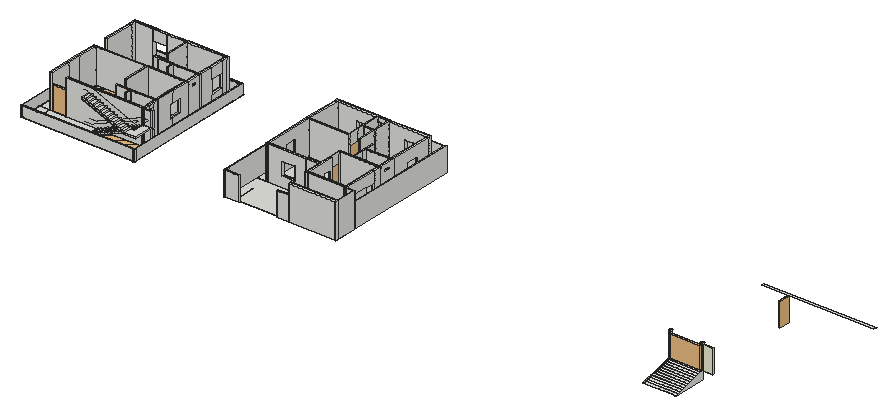
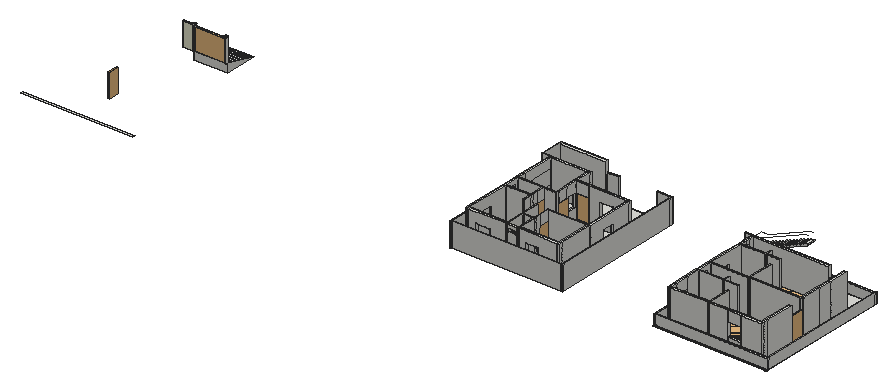
# SketchUp Ruby script. Lengths in inches.
U = 1.inch
M = Sketchup.active_model
def pt(a) = Geom::Point3d.new(a.map { |v| v * U })
def face(e, loops, mat)
  f = e.add_face(loops[0].map { |a| pt(a) })
  loops[1..].each { |l| e.add_face(l.map { |a| pt(a) }).erase! }
  f.material = f.back_material = mat if mat
  f
end
# faces: each face lists its corners as indices into pts; further lists are holes
def faces(e, pts, list, mat = nil) = list.each { |f| face(e, (f[0].is_a?(Array) ? f : [f]).map { |l| l.map { |i| pts[i] } }, mat) }
# xy, xz, yz: faces in a plane at the given z, y or x. An outline is a flat list of corners, or four numbers for a rectangle; further outlines are holes
def ring(l) = l.size == 4 ? [[l[0], l[1]], [l[2], l[1]], [l[2], l[3]], [l[0], l[3]]] : l.each_slice(2).to_a
def flat(e, list, mat, &to3) = list.each { |f| face(e, (f[0].is_a?(Array) ? f : [f]).map { |l| ring(l).map { |u, v| to3.(u, v) } }, mat) }
def xy(e, z, list, mat = nil) = flat(e, list, mat) { |x, y| [x, y, z] }
def xz(e, y, list, mat = nil) = flat(e, list, mat) { |x, z| [x, y, z] }
def yz(e, x, list, mat = nil) = flat(e, list, mat) { |y, z| [x, y, z] }
def lines(e, pts, list) = list.each { |a, b| e.add_line(pt(pts[a]), pt(pts[b])) }
# prism: a flat outline (further loops are holes) pulled along v
def prism(e, loops, v, mat = nil)
  f = face(e, loops, mat); d = Geom::Vector3d.new(v.map { |x| x * U })
  f.pushpull(f.normal.samedirection?(d) ? d.length : -d.length)
end
def box(e, o, s, mat = nil) = prism(e, [[o, [o[0] + s[0], o[1], o[2]], [o[0] + s[0], o[1] + s[1], o[2]], [o[0], o[1] + s[1], o[2]]]], [0, 0, s[2]], mat)
def at(x, y, z, deg = 0) = Geom::Transformation.translation(pt([x, y, z])) * Geom::Transformation.rotation(ORIGIN, Z_AXIS, deg.degrees)
def axes(o, x, y, z) = Geom::Transformation.new([*x, 0, *y, 0, *z, 0, *pt(o).to_a, 1])
def part(name) = M.definitions.add(name)
# library, detail: a bought-in or finely detailed component or shape, given as its bounding box
def library(name, o, s) = part(name).tap { |d| box(d.entities, o, s) }
def detail(e, o, s) = box(e.add_group.entities, o, s)
def put(e, d, t, mat = nil) = e.add_instance(d, t).tap { |i| i.material = mat if mat }
def group(e, t, mat = nil) = e.add_group.tap { |g| g.transformation = t; g.material = mat if mat }.entities
root = M.entities
M.materials.add("0001 AP 9436 AIR BREEZE").color = [243, 237, 232]
M.materials.add("0746 AP 7715 LUMINOUS").color = [235, 235, 209]
c1 = library("Group\#12",[0,0,0],[6.9375,42,86.5])
c2 = library("Group\#45",[0,0,0],[399.01,472.04,0.01])
c3 = part("Group\#29")
xy(c3.entities,0,[[0,0,0,179.49,176.02,179.49,176.02,89,180.99,89,180.99,179.49,311,179.49,311,53,176.02,53,176.02,47.99,222,47.99,222,30.01,227.01,30.01,227.01,47.99,311,47.99,311,0]])
c4 = part("Group19\#2")
p = [[1706.5625,247.76,0],[1706.5625,271.76,0],[1706.5625,427.76,65],[1706.5625,431.76,65],[1720.5625,431.76,65],[1720.5625,427.76,65],
  [1720.5625,283.76,125],[1720.5625,271.76,125],[1686.5625,247.76,0],[1686.5625,271.76,0],[1686.5625,427.76,65],[1686.5625,451.76,65],
  [1740.5625,451.76,65],[1740.5625,427.76,65],[1740.5625,283.76,125],[1740.5625,271.76,125]]
lines(c4.entities,p,[[0,1],[1,2],[2,3],[3,4],[4,5],[5,6],[6,7],[8,9],[9,10],[10,11],[11,12],[12,13],
  [13,14],[14,15]])
c5 = part("Group18\#3")
xy(c5.entities,-3.9375,[[1682.5625,271.76,1710.5625,283.76],[1682.5625,283.76,1710.5625,284.55]])
xy(c5.entities,0,[[1682.5625,271.76,1710.5625,283.76]])
xy(c5.entities,5,[[1682.5625,283.76,1710.5625,295.76]])
xy(c5.entities,10,[[1682.5625,295.76,1710.5625,307.76]])
xy(c5.entities,15,[[1682.5625,307.76,1710.5625,319.76]])
xy(c5.entities,20,[[1682.5625,319.76,1710.5625,331.76]])
xy(c5.entities,25,[[1682.5625,331.76,1710.5625,343.76]])
xy(c5.entities,30,[[1682.5625,343.76,1710.5625,355.76]])
xy(c5.entities,35,[[1682.5625,355.76,1710.5625,367.76]])
xy(c5.entities,40,[[1682.5625,367.76,1710.5625,379.76]])
xy(c5.entities,45,[[1682.5625,379.76,1710.5625,391.76]])
xy(c5.entities,50,[[1682.5625,391.76,1710.5625,403.76]])
xy(c5.entities,55,[[1682.5625,403.76,1710.5625,415.76]])
xy(c5.entities,60,[[1682.5625,415.76,1710.5625,427.76]])
xy(c5.entities,61.0625,[[1716.5625,414.97,1716.5625,427.76,1710.5625,427.76,1710.5625,440.55,1682.5625,440.55,1682.5625,455.76,1744.5625,455.76,1744.5625,414.97]])
xy(c5.entities,65,[[1716.5625,415.76,1744.5625,415.76,1744.5625,455.76,1682.5625,455.76,1682.5625,427.76,1716.5625,427.76]])
xy(c5.entities,70,[[1716.5625,403.76,1744.5625,415.76]])
xy(c5.entities,75,[[1716.5625,391.76,1744.5625,403.76]])
xy(c5.entities,80,[[1716.5625,379.76,1744.5625,391.76]])
xy(c5.entities,85,[[1716.5625,367.76,1744.5625,379.76]])
xy(c5.entities,90,[[1716.5625,355.76,1744.5625,367.76]])
xy(c5.entities,95,[[1716.5625,343.76,1744.5625,355.76]])
xy(c5.entities,100,[[1716.5625,331.76,1744.5625,343.76]])
xy(c5.entities,105,[[1716.5625,319.76,1744.5625,331.76]])
xy(c5.entities,110,[[1716.5625,307.76,1744.5625,319.76]])
xy(c5.entities,115,[[1716.5625,295.76,1744.5625,307.76]])
xy(c5.entities,120,[[1716.5625,283.76,1744.5625,295.76]])
xy(c5.entities,121.0625,[[1716.5625,270.97,1744.5625,271.76]])
xy(c5.entities,125,[[1716.5625,271.76,1744.5625,283.76]])
xz(c5.entities,271.76,[[1682.5625,-3.9375,1710.5625,0],[1716.5625,121.0625,1744.5625,125]])
xz(c5.entities,283.76,[[1682.5625,-3.9375,1710.5625,0],[1682.5625,0,1710.5625,5],[1716.5625,120,1744.5625,125]])
xz(c5.entities,295.76,[[1682.5625,5,1710.5625,10],[1716.5625,115,1744.5625,120]])
xz(c5.entities,307.76,[[1682.5625,10,1710.5625,15],[1716.5625,110,1744.5625,115]])
xz(c5.entities,319.76,[[1682.5625,15,1710.5625,20],[1716.5625,105,1744.5625,110]])
xz(c5.entities,331.76,[[1682.5625,20,1710.5625,25],[1716.5625,100,1744.5625,105]])
xz(c5.entities,343.76,[[1682.5625,25,1710.5625,30],[1716.5625,95,1744.5625,100]])
xz(c5.entities,355.76,[[1682.5625,30,1710.5625,35],[1716.5625,90,1744.5625,95]])
xz(c5.entities,367.76,[[1682.5625,35,1710.5625,40],[1716.5625,85,1744.5625,90]])
xz(c5.entities,379.76,[[1682.5625,40,1710.5625,45],[1716.5625,80,1744.5625,85]])
xz(c5.entities,391.76,[[1682.5625,45,1710.5625,50],[1716.5625,75,1744.5625,80]])
xz(c5.entities,403.76,[[1682.5625,50,1710.5625,55],[1716.5625,70,1744.5625,75]])
xz(c5.entities,415.76,[[1682.5625,55,1710.5625,60],[1716.5625,65,1744.5625,70]])
xz(c5.entities,427.76,[[1682.5625,60,1710.5625,65],[1710.5625,61.0625,1716.5625,65]])
xz(c5.entities,455.76,[[1682.5625,61.0625,1744.5625,65]])
yz(c5.entities,1682.5625,[[271.76,-3.9375,283.76,0],[283.76,-3.9375,283.76,5,295.76,5,295.76,10,307.76,10,307.76,15,319.76,15,319.76,20,331.76,20,331.76,25,343.76,25,343.76,30,355.76,30,355.76,35,367.76,35,367.76,40,379.76,40,379.76,45,391.76,45,391.76,50,403.76,50,403.76,55,415.76,55,415.76,60,427.76,60,427.76,65,455.76,65,455.76,61.0625,440.55,61.0625,284.55,-3.9375]])
yz(c5.entities,1710.5625,[[271.76,-3.9375,283.76,0],[283.76,-3.9375,284.55,-3.9375,440.55,61.0625,427.76,61.0625,427.76,60,415.76,60,415.76,55,403.76,55,403.76,50,391.76,50,391.76,45,379.76,45,379.76,40,367.76,40,367.76,35,355.76,35,355.76,30,343.76,30,343.76,25,331.76,25,331.76,20,319.76,20,319.76,15,307.76,15,307.76,10,295.76,10,295.76,5,283.76,5]])
yz(c5.entities,1716.5625,[[414.97,61.0625,270.97,121.0625,271.76,121.0625,271.76,125,283.76,125,283.76,120,295.76,120,295.76,115,307.76,115,307.76,110,319.76,110,319.76,105,331.76,105,331.76,100,343.76,100,343.76,95,355.76,95,355.76,90,367.76,90,367.76,85,379.76,85,379.76,80,391.76,80,391.76,75,403.76,75,403.76,70,415.76,70,415.76,65,427.76,65,427.76,61.0625]])
yz(c5.entities,1744.5625,[[414.97,61.0625,455.76,61.0625,455.76,65,415.76,65,415.76,70,403.76,70,403.76,75,391.76,75,391.76,80,379.76,80,379.76,85,367.76,85,367.76,90,355.76,90,355.76,95,343.76,95,343.76,100,331.76,100,331.76,105,319.76,105,319.76,110,307.76,110,307.76,115,295.76,115,295.76,120,283.76,120,283.76,125,271.76,125,271.76,121.0625,270.97,121.0625]])
p = [[1682.5625,284.55,-3.9375],[1682.5625,440.55,61.0625],[1710.5625,440.55,61.0625],[1710.5625,284.55,-3.9375],[1744.5625,414.97,61.0625],[1744.5625,270.97,121.0625],
  [1716.5625,270.97,121.0625],[1716.5625,414.97,61.0625]]
faces(c5.entities,p,[[0,1,2,3],[4,5,6,7]])
put(c5.entities,c4,at(0,0,24))
c6 = library("Group\#65",[0,0,0],[128.92,12.7,76.26])
box(root,[369.99,129.92,0],[24.01,2.89,120])
xy(root,-0.68,[[2163.39,584.56,2555.38,593.76]])
xy(root,-0.22,[[2327.68,112.52,2333.68,118.52]])
xy(root,0,[[1097.625,52.39,1102.64,130.94],[1097.625,130.94,1102.64,133.92],[1011.11,277.13,1047.11,277.22,1047.11,277.35,1011.11,277.26]])
xy(root,0.29,[[2216.4,112.52,2222.4,118.52]])
xy(root,83.78,[[[2326.68,111.52,2334.68,119.52],[2327.68,112.52,2333.68,118.52]]])
xy(root,84.29,[[[2215.4,111.52,2223.4,119.52],[2216.4,112.52,2222.4,118.52]]])
xy(root,84.38,[[[2326.68,111.52,2334.68,119.52],[2327.68,112.52,2333.68,118.52]]])
xy(root,84.68,[[2327.68,112.52,2333.68,118.52]])
xy(root,84.89,[[[2215.4,111.52,2223.4,119.52],[2216.4,112.52,2222.4,118.52]]])
xy(root,85.19,[[2216.4,112.52,2222.4,118.52]])
xy(root,120,[[1097.625,52.39,1102.64,130.94],[1075.625,129.92,1097.625,129.92,1097.625,130.94,1102.64,130.94,1102.64,133.92,1075.625,133.92]])
xz(root,52.39,[[1097.625,0,1102.64,120]])
xz(root,111.52,[[2326.68,83.78,2334.68,84.38],[2215.4,84.29,2223.4,84.89]])
xz(root,112.52,[[2327.68,-0.22,2333.68,83.78],[2216.4,0.29,2222.4,84.29],[2327.68,83.78,2333.68,84.38],[2216.4,84.29,2222.4,84.89],[2327.68,84.38,2333.68,84.68],
  [2216.4,84.89,2222.4,85.19]])
xz(root,118.52,[[2327.68,-0.22,2333.68,83.78],[2216.4,0.29,2222.4,84.29],[2327.68,83.78,2333.68,84.38],[2216.4,84.29,2222.4,84.89],[2327.68,84.38,2333.68,84.68],
  [2216.4,84.89,2222.4,85.19]])
xz(root,119.52,[[2326.68,83.78,2334.68,84.38],[2215.4,84.29,2223.4,84.89]])
xz(root,129.92,[[1075.625,0,1097.625,120]])
xz(root,130.94,[[1097.625,0,1102.64,120]])
xz(root,133.92,[[1075.625,0,1102.64,120]])
yz(root,1075.625,[[129.92,0,133.92,120]])
yz(root,1097.625,[[52.39,0,129.92,120],[129.92,0,130.94,120]])
yz(root,1102.64,[[52.39,0,61.42,120],[61.42,0,130.94,120],[130.94,0,133.92,120]])
yz(root,2215.4,[[111.52,84.29,119.52,84.89]])
yz(root,2216.4,[[112.52,0.29,118.52,84.29],[112.52,84.29,118.52,84.89],[112.52,84.89,118.52,85.19]])
yz(root,2222.4,[[112.52,0.29,118.52,84.29],[112.52,84.29,118.52,84.89],[112.52,84.89,118.52,85.19]])
yz(root,2223.4,[[111.52,84.29,119.52,84.89]])
yz(root,2326.68,[[111.52,83.78,119.52,84.38]])
yz(root,2327.68,[[112.52,-0.22,118.52,83.78],[112.52,83.78,118.52,84.38],[112.52,84.38,118.52,84.68]])
yz(root,2333.68,[[112.52,-0.22,118.52,83.78],[112.52,83.78,118.52,84.38],[112.52,84.38,118.52,84.68]])
yz(root,2334.68,[[111.52,83.78,119.52,84.38]])
p = [[930.07,127.77,0],[930.33,99.77,0],[930.33,99.77,3.9375],[930.07,127.77,3.9375]]
faces(root,p,[[0,1,2,3]])
put(root,c1,axes([41.43,323.41,0],[0.85622,0,0],[0,1.14256,0],[0,0,0.9711]))
put(root,c1,axes([98.03,130.35,0],[0,0.89531,0],[-1.14256,0,0],[0,0,0.9711]))
put(root,c2,at(0,52.39,0))
g1 = group(root,at(5.01,500.42,0))
xy(g1,0,[[0,-443.02,36,-370.5],[36,-443.02,200.49,-370.5],[0,-370.5,36,0],[200.49,-370.5,364.98,-367.61],[364.98,-367.61,388.99,0],
  [0,0,364.98,19.01],[364.98,0,388.99,19.01]])
xy(g1,1,[[0,-443.02,36,-370.5],[36,-443.02,200.49,-370.5],[0,-370.5,36,0],[200.49,-370.5,364.98,-367.61],[364.98,-367.61,388.99,0],
  [0,0,364.98,19.01],[364.98,0,388.99,19.01]])
xz(g1,-443.02,[[0,0,36,1],[36,0,200.49,1]])
xz(g1,-370.5,[[0,0,36,1],[36,0,364.98,1]])
xz(g1,-367.61,[[200.49,0,388.99,1]])
xz(g1,0,[[0,0,36,1],[36,0,364.98,1],[364.98,0,388.99,1]])
xz(g1,19.01,[[0,0,364.98,1],[364.98,0,388.99,1]])
yz(g1,0,[[-443.02,0,-370.5,1],[-370.5,0,0,1],[0,0,19.01,1]])
yz(g1,36,[[-443.02,0,-370.5,1],[-370.5,0,0,1]])
yz(g1,200.49,[[-443.02,0,-367.61,1]])
yz(g1,364.98,[[-370.5,0,0,1],[0,0,19.01,1]])
yz(g1,388.99,[[-367.61,0,0,1],[0,0,19.01,1]])
g2 = group(root,at(0,512.6,0))
xy(g2,0,[[0,-460.21,5.01,-455.2],[5.01,-460.21,394,-455.2],[394,-460.21,399.01,-455.2],[0,-455.2,5.01,6.82],[394,-455.2,399.01,11.83],
  [0,6.82,394,11.83]])
xy(g2,36,[[0,-460.21,5.01,-455.2],[5.01,-460.21,394,-455.2],[394,-460.21,399.01,-455.2],[0,-455.2,5.01,6.82],[394,-455.2,399.01,11.83],
  [0,6.82,394,11.83]])
xz(g2,-460.21,[[0,0,5.01,36],[5.01,0,394,36],[394,0,399.01,36]])
xz(g2,-455.2,[[0,0,5.01,36],[5.01,0,394,36]])
xz(g2,6.82,[[0,0,5.01,36],[5.01,0,394,36]])
xz(g2,11.83,[[0,0,394,36],[394,0,399.01,36]])
yz(g2,0,[[-460.21,0,-455.2,36],[-455.2,0,6.82,36],[6.82,0,11.83,36]])
yz(g2,5.01,[[-460.21,0,-455.2,36],[-455.2,0,6.82,36]])
yz(g2,394,[[-460.21,0,-455.2,36],[-455.2,0,6.82,36],[6.82,0,11.83,36]])
yz(g2,399.01,[[-460.21,0,-455.2,36],[-455.2,0,11.83,36]])
put(root,c2,at(0,56.39,0))
g3 = group(root,at(41.01,475.65,0))
xy(g3,0,[[0,-345.73,8.99,-275.49],[57.02,-345.73,319.99,-336.74],[319.99,-345.73,328.98,-336.74],[319.99,-336.74,328.98,-321.76],[319.99,-321.76,328.98,-303.74],
  [230.99,-306.73,236,-288.76],[319.99,-303.74,328.98,-288.76],[185.01,-288.76,230.99,-283.75],[230.99,-288.76,236,-283.75],[236,-288.76,236.3,-283.75],
  [236.3,-288.76,319.99,-283.75],[319.99,-288.76,328.98,-283.75],[319.99,-283.75,328.98,-220.31],[0,-275.49,8.99,-227.5],[185.01,-247.75,189.98,-157.25],
  [0,-227.5,8.99,-157.25],[319.99,-220.31,328.98,-152.24],[0,-157.25,8.99,-152.24],[8.99,-157.25,185.01,-152.24],[185.01,-157.25,189.98,-152.24],
  [189.98,-157.25,319.99,-152.24],[8.99,-152.24,8.99,15.78,185.01,15.78,185.01,-63.24,189.98,-63.24,189.98,15.78,319.99,15.78,319.99,-99.25,185.01,-99.25,185.01,-104.25,230.99,-104.25,230.99,-122.23,236,-122.23,236,-104.25,319.99,-104.25,319.99,-152.24],[319.99,-152.24,328.98,-104.25],[230.99,-122.23,236,-104.25],[0,-104.25,8.99,0],
  [185.01,-104.25,230.99,-99.25],[230.99,-104.25,236,-99.25],[236,-104.25,319.99,-99.25],[319.99,-104.25,328.98,-99.25],[319.99,-99.25,328.98,-51.73],
  [185.01,-63.24,189.98,15.78],[319.99,-51.73,328.98,-3.7],[319.99,-3.7,328.98,15.78],[0,0,8.99,15.78],[0,15.78,71.96,24.77],
  [71.96,15.78,119.95,24.77],[119.95,15.78,185.01,24.77],[185.01,15.78,189.98,24.77],[189.98,15.78,319.99,24.77],[319.99,15.78,328.98,24.77]])
xy(g3,36,[[319.99,-233.25,328.98,-185.25],[319.99,-51.73,328.98,-3.7],[71.96,15.78,119.95,24.77]])
xy(g3,84,[[319.99,-233.25,328.98,-185.25],[319.99,-51.73,328.98,-3.7],[71.96,15.78,119.95,24.77]])
xy(g3,95.92,[[319.99,-138.12,328.98,-118.25]])
xy(g3,96,[[319.99,-321.76,328.98,-303.74]])
xy(g3,108,[[319.99,-321.76,328.98,-303.74]])
xy(g3,108.21,[[319.99,-138.12,328.98,-118.25]])
xy(g3,120,[[0,-345.73,8.99,-275.49],[57.02,-345.73,319.99,-336.74],[319.99,-345.73,328.98,-336.74],[319.99,-336.74,328.98,-321.76],[319.99,-321.76,328.98,-303.74],
  [230.99,-306.73,236,-288.76],[319.99,-303.74,328.98,-288.76],[185.01,-288.76,230.99,-283.75],[230.99,-288.76,236,-283.75],[236,-288.76,236.3,-283.75],
  [236.3,-288.76,319.99,-283.75],[319.99,-288.76,328.98,-283.75],[319.99,-283.75,328.98,-220.31],[0,-275.49,8.99,-227.5],[185.01,-247.75,189.98,-157.25],
  [0,-227.5,8.99,-157.25],[319.99,-220.31,328.98,-152.24],[0,-157.25,8.99,-152.24],[8.99,-157.25,185.01,-152.24],[185.01,-157.25,189.98,-152.24],
  [189.98,-157.25,319.99,-152.24],[319.99,-152.24,328.98,-104.25],[230.99,-122.23,236,-104.25],[0,-104.25,8.99,0],[185.01,-104.25,230.99,-99.25],
  [230.99,-104.25,236,-99.25],[236,-104.25,319.99,-99.25],[319.99,-104.25,328.98,-99.25],[319.99,-99.25,328.98,-51.73],[185.01,-63.24,189.98,15.78],
  [319.99,-51.73,328.98,-3.7],[319.99,-3.7,328.98,15.78],[0,0,8.99,15.78],[0,15.78,71.96,24.77],[71.96,15.78,119.95,24.77],
  [119.95,15.78,185.01,24.77],[185.01,15.78,189.98,24.77],[189.98,15.78,319.99,24.77],[319.99,15.78,328.98,24.77]])
xz(g3,-345.73,[[0,0,8.99,120],[57.02,0,319.99,120],[319.99,0,328.98,120]])
xz(g3,-336.74,[[57.02,0,319.99,120],[319.99,0,328.98,120]])
xz(g3,-321.76,[[319.99,0,328.98,96],[319.99,96,328.98,108],[319.99,108,328.98,120]])
xz(g3,-306.73,[[230.99,0,236,120]])
xz(g3,-303.74,[[319.99,0,328.98,96],[319.99,96,328.98,108],[319.99,108,328.98,120]])
xz(g3,-288.76,[[185.01,0,230.99,120],[230.99,0,236,120],[236,0,236.3,120],[236.3,0,319.99,120],[319.99,0,328.98,120]])
xz(g3,-283.75,[[185.01,0,230.99,120],[230.99,0,236,120],[236,0,236.3,120],[236.3,0,319.99,120],[319.99,0,328.98,120]])
xz(g3,-275.49,[[0,0,8.99,120]])
xz(g3,-247.75,[[185.01,0,189.98,120]])
xz(g3,-233.25,[[319.99,36,328.98,84]])
xz(g3,-227.5,[[0,0,8.99,120]])
xz(g3,-185.25,[[319.99,36,328.98,84]])
xz(g3,-157.25,[[0,0,8.99,120],[8.99,0,185.01,120],[185.01,0,189.98,120],[189.98,0,319.99,120]])
xz(g3,-152.24,[[0,0,8.99,120],[8.99,0,185.01,120],[185.01,0,189.98,120],[189.98,0,319.99,120],[319.99,0,328.98,120]])
xz(g3,-138.12,[[319.99,95.92,328.98,108.21]])
xz(g3,-122.23,[[230.99,0,236,120]])
xz(g3,-118.25,[[319.99,95.92,328.98,108.21]])
xz(g3,-104.25,[[0,0,8.99,120],[185.01,0,230.99,120],[230.99,0,236,120],[236,0,319.99,120],[319.99,0,328.98,120]])
xz(g3,-99.25,[[185.01,0,230.99,120],[230.99,0,236,120],[236,0,319.99,120],[319.99,0,328.98,120]])
xz(g3,-63.24,[[185.01,0,189.98,120]])
xz(g3,-51.73,[[319.99,0,328.98,36],[319.99,36,328.98,84],[319.99,84,328.98,120]])
xz(g3,-3.7,[[319.99,0,328.98,36],[319.99,36,328.98,84],[319.99,84,328.98,120]])
xz(g3,0,[[0,0,8.99,120]])
xz(g3,15.78,[[0,0,8.99,120],[8.99,0,71.96,120],[71.96,0,119.95,36],[119.95,0,185.01,120],[185.01,0,189.98,120],
  [189.98,0,319.99,120],[319.99,0,328.98,120],[71.96,84,119.95,120]])
xz(g3,24.77,[[0,0,71.96,120],[71.96,0,119.95,36],[119.95,0,185.01,120],[185.01,0,189.98,120],[189.98,0,319.99,120],
  [319.99,0,328.98,120],[71.96,84,119.95,120]])
yz(g3,0,[[-345.73,0,-275.49,120],[-275.49,0,-227.5,120],[-227.5,0,-157.25,120],[-157.25,0,-152.24,120],[-104.25,0,0,120],
  [0,0,15.78,120],[15.78,0,24.77,120]])
yz(g3,8.99,[[-345.73,0,-275.49,120],[-275.49,0,-227.5,120],[-227.5,0,-157.25,120],[-157.25,0,-152.24,120],[-104.25,0,0,120],
  [0,0,15.78,120]])
yz(g3,57.02,[[-345.73,0,-336.74,120]])
yz(g3,71.96,[[15.78,0,24.77,36],[15.78,36,24.77,84],[15.78,84,24.77,120]])
yz(g3,119.95,[[15.78,0,24.77,36],[15.78,36,24.77,84],[15.78,84,24.77,120]])
yz(g3,185.01,[[-288.76,0,-283.75,120],[-247.75,0,-157.25,120],[-157.25,0,-152.24,120],[-104.25,0,-99.25,120],[-63.24,0,15.78,120],
  [15.78,0,24.77,120]])
yz(g3,189.98,[[-247.75,0,-157.25,120],[-157.25,0,-152.24,120],[-63.24,0,15.78,120],[15.78,0,24.77,120]])
yz(g3,230.99,[[-306.73,0,-288.76,120],[-288.76,0,-283.75,120],[-122.23,0,-104.25,120],[-104.25,0,-99.25,120]])
yz(g3,236,[[-306.73,0,-288.76,120],[-288.76,0,-283.75,120],[-122.23,0,-104.25,120],[-104.25,0,-99.25,120]])
yz(g3,236.3,[[-288.76,0,-283.75,120]])
yz(g3,319.99,[[-345.73,0,-336.74,120],[-336.74,0,-321.76,120],[-321.76,0,-303.74,96],[-303.74,0,-288.76,120],[-288.76,0,-283.75,120],
  [[-283.75,0,-157.25,120],[-233.25,36,-185.25,84]],[-157.25,0,-152.24,120],[[-152.24,0,-104.25,120],[-138.12,95.92,-118.25,108.21]],[-104.25,0,-99.25,120],[-99.25,0,-51.73,120],
  [-51.73,0,-3.7,36],[-3.7,0,15.78,120],[15.78,0,24.77,120],[-51.73,84,-3.7,120],[-321.76,108,-303.74,120]])
yz(g3,328.98,[[-345.73,0,-336.74,120],[-336.74,0,-321.76,120],[-321.76,0,-303.74,96],[-303.74,0,-288.76,120],[-288.76,0,-283.75,120],
  [-283.75,0,-220.31,0,-220.31,36,-233.25,36,-233.25,84,-220.31,84,-220.31,120,-283.75,120],[-220.31,0,-152.24,0,-152.24,120,-220.31,120,-220.31,84,-185.25,84,-185.25,36,-220.31,36],[[-152.24,0,-104.25,120],[-138.12,95.92,-118.25,108.21]],[-104.25,0,-99.25,120],[-99.25,0,-51.73,120],
  [-51.73,0,-3.7,36],[-3.7,0,15.78,120],[15.78,0,24.77,120],[-51.73,84,-3.7,120],[-321.76,108,-303.74,120]])
put(g3,c3,at(8.99,-336.74,0))
put(root,c1,axes([271,323.41,0],[0.86547,0,0],[0,0.71448,0],[0,0,0.9711]))
put(root,c1,axes([271.06,138.91,0],[0.85748,0,0],[0,0.71448,0],[0,0,0.9711]))
put(root,c5,axes([-83.12,1973.1875,3.98],[0.01009,-1.09803,0],[1.00962,0.00928,0],[0,0,1.01]))
put(root,c1,axes([896.94,407.27,0],[-0.90684,0,0],[0,-0.85428,0],[0,0,0.9711]))
g4 = group(root,at(715.65,493.16,0))
xy(g4,0,[[0,-435.76,0,-304.77,215.96,-304.77,215.96,-359.24,30.99,-359.24,30.99,-435.76],[30.99,-435.76,381.97,-359.24],[359.97,-359.24,381.97,7.26],[0,-304.77,30.99,0],[0,0,30.99,7.26],
  [0,7.26,30.99,35.34],[30.99,7.26,359.97,35.34],[359.97,7.26,381.97,35.34]])
xy(g4,1,[[0,-435.76,381.97,-435.76,381.97,-359.24,215.96,-359.24,215.96,-304.77,0,-304.77],[359.97,-359.24,381.97,7.26],[0,-304.77,30.99,0],[0,0,30.99,7.26],[0,7.26,30.99,35.34],
  [30.99,7.26,359.97,35.34],[359.97,7.26,381.97,35.34]])
xz(g4,-435.76,[[0,0,30.99,1],[30.99,0,381.97,1]])
xz(g4,-359.24,[[215.96,0,359.97,1]])
xz(g4,-304.77,[[0,0,30.99,1],[30.99,0,215.96,1]])
xz(g4,0,[[0,0,30.99,1]])
xz(g4,7.26,[[0,0,30.99,1],[30.99,0,359.97,1],[359.97,0,381.97,1]])
xz(g4,35.34,[[0,0,30.99,1],[30.99,0,359.97,1],[359.97,0,381.97,1]])
yz(g4,0,[[-435.76,0,-304.77,1],[-304.77,0,0,1],[0,0,7.26,1],[7.26,0,35.34,1]])
yz(g4,30.99,[[-435.76,0,-359.24,1],[-304.77,0,0,1],[0,0,7.26,1],[7.26,0,35.34,1]])
yz(g4,215.96,[[-359.24,0,-304.77,1]])
yz(g4,359.97,[[-359.24,0,7.26,1],[7.26,0,35.34,1]])
yz(g4,381.97,[[-435.76,0,-359.24,1],[-359.24,0,7.26,1],[7.26,0,35.34,1]])
g5 = group(root,at(710.65,518.89,0))
xy(g5,0,[[0,-466.5,5.01,-461.49],[5.01,-466.5,53.01,-461.49],[0,-461.49,5.01,-452.29],[0,-452.29,5.01,9.73],[386.98,-384.97,391.99,14.74],
  [0,9.73,5.01,14.74],[5.01,9.73,386.98,14.74]])
xy(g5,84,[[0,-466.5,5.01,-461.49],[5.01,-466.5,53.01,-461.49],[0,-461.49,5.01,-452.29],[0,-452.29,5.01,9.73],[386.98,-384.97,391.99,14.74],
  [0,9.73,5.01,14.74],[5.01,9.73,386.98,14.74]])
xz(g5,-466.5,[[0,0,5.01,84],[5.01,0,53.01,84]])
xz(g5,-461.49,[[0,0,5.01,84],[5.01,0,53.01,84]])
xz(g5,-452.29,[[0,0,5.01,84]])
xz(g5,-384.97,[[386.98,0,391.99,84]])
xz(g5,9.73,[[0,0,5.01,84],[5.01,0,386.98,84]])
xz(g5,14.74,[[0,0,5.01,84],[5.01,0,386.98,84],[386.98,0,391.99,84]])
yz(g5,0,[[-466.5,0,-461.49,84],[-461.49,0,-452.29,84],[-452.29,0,9.73,84],[9.73,0,14.74,84]])
yz(g5,5.01,[[-466.5,0,-461.49,84],[-461.49,0,-452.29,84],[-452.29,0,9.73,84],[9.73,0,14.74,84]])
yz(g5,53.01,[[-466.5,0,-461.49,84]])
yz(g5,386.98,[[-384.97,0,9.73,84],[9.73,0,14.74,84]])
yz(g5,391.99,[[-384.97,0,14.74,84]])
put(root,c1,axes([931.62,188.99,0],[0,0.7279,0],[-1.06713,0,0],[0,0,0.9711]))
g6 = group(root,at(746.65,491.43,0))
xy(g6,0,[[184.97,-361.51,194,-352.52],[194,-361.51,319.99,-352.52],[319.99,-361.51,328.98,-352.52],[184.97,-352.52,194,-303.04],[194,-352.52,319.99,-303.04],
  [319.99,-352.52,328.98,-303.04],[0,-303.04,8.99,-294.03],[8.99,-303.04,140.15,-294.03],[184.97,-303.04,194,-253.68],[319.99,-303.04,328.98,-238.48],
  [0,-294.03,8.99,-294],[0,-294,8.99,-125],[319.99,-238.48,328.98,-214.09],[184.97,-218.02,189.98,-214.09],[184.97,-214.09,189.98,-209.03],
  [189.98,-214.09,319.99,-209.03],[319.99,-214.09,328.98,-209.03],[319.99,-209.03,328.98,-155.01],[230.99,-179.02,236,-160.01],[230.99,-160.01,236,-155.01],
  [236,-160.01,319.99,-155.01],[230.99,-155.01,236,-125],[319.99,-155.01,328.98,0],[0,-125,8.99,-120.03],[8.99,-125,148.97,-120.03],
  [184.97,-125,189.98,-65.02],[0,-120.03,8.99,0],[144,-84.03,148.97,-65.02],[144,-65.02,148.97,-60.02],[148.97,-65.02,151.97,-60.02],
  [181.98,-65.02,184.97,-60.02],[184.97,-65.02,189.98,-60.02],[144,-60.02,148.97,0],[184.97,-60.02,189.98,0],[0,0,8.99,8.99],
  [8.99,0,144,8.99],[144,0,148.97,8.99],[148.97,0,184.97,8.99],[184.97,0,189.98,8.99],[189.98,0,319.99,8.99],
  [319.99,0,328.98,8.99]])
xy(g6,36,[[319.99,-352.52,328.98,-274.28],[55.86,-303.04,103.86,-294.03],[319.99,-274.28,328.98,-238.48],[0,-225,8.99,-179.55],[319.99,-96,328.98,-48],
  [77.49,0,118.65,8.99],[244.5,0,291.95,8.99]])
xy(g6,36.59,[[184.97,-290.84,194,-258.52]])
xy(g6,83.83,[[0,-225,8.99,-179.55]])
xy(g6,83.9,[[77.49,0,118.65,8.99]])
xy(g6,84,[[319.99,-352.52,328.98,-274.28],[55.86,-303.04,103.86,-294.03],[140.15,-303.04,184.97,-294.03],[319.99,-274.28,328.98,-238.48],[184.97,-253.68,189.49,-218.02],
  [230.99,-209.03,236.12,-179.02],[144,-120.03,148.97,-84.03],[319.99,-96,328.98,-48],[151.97,-65.02,181.98,-60.02],[244.5,0,291.95,8.99]])
xy(g6,85.87,[[184.97,-290.84,194,-258.52]])
xy(g6,96,[[319.99,-197.03,328.98,-172.01],[154.97,0,178.97,8.99]])
xy(g6,108,[[319.99,-197.03,328.98,-172.01],[154.97,0,178.97,8.99]])
xy(g6,120,[[184.97,-361.51,194,-352.52],[194,-361.51,319.99,-352.52],[319.99,-361.51,328.98,-352.52],[184.97,-352.52,194,-253.68],[319.99,-352.52,328.98,-238.48],
  [0,-303.04,8.99,-294.03],[8.99,-303.04,140.15,-294.03],[140.15,-303.04,184.97,-294.03],[0,-294.03,8.99,-294],[0,-294,8.99,-125],
  [184.97,-253.68,189.49,-218.02],[319.99,-238.48,328.98,-214.09],[184.97,-218.02,189.98,-214.09],[184.97,-214.09,189.98,-209.03],[189.98,-214.09,319.99,-209.03],
  [319.99,-214.09,328.98,-209.03],[230.99,-209.03,236.12,-179.02],[319.99,-209.03,328.98,-155.01],[230.99,-179.02,236,-160.01],[230.99,-160.01,236,-155.01],
  [236,-160.01,319.99,-155.01],[230.99,-155.01,236,-125],[319.99,-155.01,328.98,0],[0,-125,8.99,-120.03],[8.99,-125,148.97,-120.03],
  [184.97,-125,189.98,-65.02],[0,-120.03,8.99,0],[144,-120.03,148.97,-84.03],[144,-84.03,148.97,-65.02],[144,-65.02,148.97,-60.02],
  [148.97,-65.02,151.97,-60.02],[151.97,-65.02,181.98,-60.02],[181.98,-65.02,184.97,-60.02],[184.97,-65.02,189.98,-60.02],[144,-60.02,148.97,0],
  [184.97,-60.02,189.98,0],[0,0,8.99,8.99],[8.99,0,144,8.99],[144,0,148.97,8.99],[148.97,0,184.97,8.99],
  [184.97,0,189.98,8.99],[189.98,0,319.99,8.99],[319.99,0,328.98,8.99]])
xz(g6,-361.51,[[184.97,0,194,120],[194,0,319.99,120],[319.99,0,328.98,120]])
xz(g6,-352.52,[[184.97,0,194,120],[194,0,319.99,120],[319.99,0,328.98,36],[319.99,84,328.98,120]])
xz(g6,-303.04,[[0,0,8.99,120],[[8.99,0,140.15,120],[55.86,36,103.86,84]],[140.15,84,184.97,120]])
xz(g6,-294.03,[[0,0,8.99,120],[[8.99,0,140.15,120],[55.86,36,103.86,84]],[140.15,84,184.97,120]])
xz(g6,-294,[[0,0,8.99,120]])
xz(g6,-290.84,[[184.97,36.59,194,85.87]])
xz(g6,-274.28,[[319.99,36,328.98,84]])
xz(g6,-258.52,[[184.97,36.59,194,85.87]])
xz(g6,-253.68,[[184.97,0,184.97,84,189.49,84,189.49,120,194,120,194,0],[184.97,84,189.49,120]])
xz(g6,-238.48,[[319.99,0,328.98,36],[319.99,36,328.98,84],[319.99,84,328.98,120]])
xz(g6,-225,[[0,36,8.99,83.83]])
xz(g6,-218.02,[[184.97,0,189.98,0,189.98,120,189.49,120,189.49,84,184.97,84],[184.97,84,189.49,120]])
xz(g6,-214.09,[[184.97,0,189.98,120],[189.98,0,319.99,120],[319.99,0,328.98,120]])
xz(g6,-209.03,[[184.97,0,189.98,120],[189.98,0,189.98,120,230.99,120,230.99,84,236.12,84,236.12,120,319.99,120,319.99,0],[319.99,0,328.98,120],[230.99,84,236.12,120]])
xz(g6,-197.03,[[319.99,96,328.98,108]])
xz(g6,-179.55,[[0,36,8.99,83.83]])
xz(g6,-179.02,[[230.99,0,236,84],[230.99,84,236,120],[236,84,236.12,120]])
xz(g6,-172.01,[[319.99,96,328.98,108]])
xz(g6,-160.01,[[230.99,0,236,120],[236,0,319.99,120]])
xz(g6,-155.01,[[230.99,0,236,120],[236,0,319.99,120],[319.99,0,328.98,120]])
xz(g6,-125,[[0,0,8.99,120],[8.99,0,148.97,120],[184.97,0,189.98,120],[230.99,0,236,120]])
xz(g6,-120.03,[[0,0,8.99,120],[8.99,0,8.99,120,144,120,144,84,148.97,84,148.97,0],[144,84,148.97,120]])
xz(g6,-96,[[319.99,36,328.98,84]])
xz(g6,-84.03,[[144,0,148.97,84],[144,84,148.97,120]])
xz(g6,-65.02,[[144,0,148.97,120],[148.97,0,151.97,120],[181.98,0,184.97,120],[184.97,0,189.98,120],[151.97,84,181.98,120]])
xz(g6,-60.02,[[144,0,148.97,120],[148.97,0,151.97,120],[181.98,0,184.97,120],[184.97,0,189.98,120],[151.97,84,181.98,120]])
xz(g6,-48,[[319.99,36,328.98,84]])
xz(g6,0,[[0,0,8.99,120],[[8.99,0,144,120],[77.49,36,118.65,83.9]],[144,0,148.97,120],[[148.97,0,184.97,120],[154.97,96,178.97,108]],[184.97,0,189.98,120],
  [[189.98,0,319.99,120],[244.5,36,291.95,84]],[319.99,0,328.98,120]])
xz(g6,8.99,[[0,0,8.99,120],[[8.99,0,144,120],[77.49,36,118.65,83.9]],[144,0,148.97,120],[[148.97,0,184.97,120],[154.97,96,178.97,108]],[184.97,0,189.98,120],
  [[189.98,0,319.99,120],[244.5,36,291.95,84]],[319.99,0,328.98,120]])
yz(g6,0,[[-303.04,0,-294.03,120],[-294.03,0,-294,120],[[-294,0,-125,120],[-225,36,-179.55,83.83]],[-125,0,-120.03,120],[-120.03,0,0,120],
  [0,0,8.99,120]])
yz(g6,8.99,[[-303.04,0,-294.03,120],[-294.03,0,-294,120],[[-294,0,-125,120],[-225,36,-179.55,83.83]],[-125,0,-120.03,120],[-120.03,0,0,120],
  [0,0,8.99,120]])
yz(g6,55.86,[[-303.04,36,-294.03,84]])
yz(g6,77.49,[[0,36,8.99,83.9]])
yz(g6,103.86,[[-303.04,36,-294.03,84]])
yz(g6,118.65,[[0,36,8.99,83.9]])
yz(g6,140.15,[[-303.04,0,-294.03,84],[-303.04,84,-294.03,120]])
yz(g6,144,[[-84.03,0,-65.02,120],[-65.02,0,-60.02,120],[-60.02,0,0,120],[0,0,8.99,120],[-120.03,84,-84.03,120]])
yz(g6,148.97,[[-125,0,-120.03,120],[-84.03,0,-65.02,120],[-65.02,0,-60.02,120],[-60.02,0,0,120],[0,0,8.99,120],
  [-120.03,84,-84.03,120]])
yz(g6,151.97,[[-65.02,0,-60.02,84],[-65.02,84,-60.02,120]])
yz(g6,154.97,[[0,96,8.99,108]])
yz(g6,178.97,[[0,96,8.99,108]])
yz(g6,181.98,[[-65.02,0,-60.02,84],[-65.02,84,-60.02,120]])
yz(g6,184.97,[[-361.51,0,-352.52,120],[[-352.52,0,-352.52,120,-303.04,120,-303.04,84,-294.03,84,-294.03,120,-253.68,120,-253.68,0],[-290.84,36.59,-258.52,85.87]],[-218.02,0,-214.09,120],[-214.09,0,-209.03,120],[-125,0,-65.02,120],
  [-65.02,0,-60.02,120],[-60.02,0,0,120],[0,0,8.99,120],[-303.04,84,-294.03,120],[-253.68,84,-218.02,120]])
yz(g6,189.49,[[-253.68,84,-218.02,120]])
yz(g6,189.98,[[-218.02,0,-214.09,120],[-214.09,0,-209.03,120],[-125,0,-65.02,120],[-65.02,0,-60.02,120],[-60.02,0,0,120],
  [0,0,8.99,120]])
yz(g6,194,[[-361.51,0,-352.52,120],[[-352.52,0,-253.68,120],[-290.84,36.59,-258.52,85.87]]])
yz(g6,230.99,[[-179.02,0,-160.01,120],[-160.01,0,-155.01,120],[-155.01,0,-125,120],[-209.03,84,-179.02,120]])
yz(g6,236,[[-179.02,0,-160.01,120],[-160.01,0,-155.01,120],[-155.01,0,-125,120]])
yz(g6,236.12,[[-209.03,84,-179.02,120]])
yz(g6,244.5,[[0,36,8.99,84]])
yz(g6,291.95,[[0,36,8.99,84]])
yz(g6,319.99,[[-361.51,0,-352.52,120],[-352.52,0,-280.02,36],[-280.02,0,-238.48,36],[-238.48,0,-214.09,120],[-214.09,0,-209.03,120],
  [[-209.03,0,-160.01,120],[-197.03,96,-172.01,108]],[-160.01,0,-155.01,120],[[-155.01,0,0,120],[-96,36,-48,84]],[0,0,8.99,120],[-352.52,36,-274.28,84],
  [-352.52,84,-238.48,120]])
yz(g6,328.98,[[-361.51,0,-352.52,0,-352.52,36,-274.28,36,-274.28,84,-352.52,84,-352.52,120,-361.51,120],[-352.52,0,-238.48,36],[-238.48,0,-214.09,120],[-214.09,0,-209.03,120],[[-209.03,0,-155.01,120],[-197.03,96,-172.01,108]],
  [[-155.01,0,0,120],[-96,36,-48,84]],[0,0,8.99,120],[-352.52,84,-238.48,120]])
# 2 loose lines left out
g7 = group(g6,at(8.99,-303.04,0))
xy(g7,0,[[131.16,0,131.16,9.01,0,9.01,0,178.04,139.98,178.04,139.98,183,0,183,0,303.04,135.02,303.04,135.02,219,139.98,219,139.98,238.01,142.98,238.01,142.98,243.02,139.98,243.02,139.98,303.04,175.98,303.04,175.98,243.02,172.99,243.02,172.99,238.01,175.98,238.01,175.98,178.04,180.99,178.04,180.99,303.04,311,303.04,311,148.03,227.01,148.03,227.01,178.04,222,178.04,222,124.01,227.01,124.01,227.01,143.02,311,143.02,311,94.01,175.98,94.01,175.98,85.02,180.99,85.02,180.99,88.95,311,88.95,311,0,185.01,0,185.01,49.36,175.98,49.36,175.98,0]])
put(root,c1,axes([929.32,426.36,0],[0,0.7279,0],[-0.73015,0,0],[0,0,0.9711]))
g8 = group(root,at(928.52,52.39,0))
xy(g8,0,[[-32,0,8.1,5.01]])
xy(g8,84,[[-32,0,8.1,5.01]])
xz(g8,0,[[-32,0,8.1,84]])
xz(g8,5.01,[[-32,0,8.1,84]])
yz(g8,-32,[[0,0,5.01,84]])
yz(g8,8.1,[[0,0,5.01,84]])
put(root,c1,axes([930.2,237.75,0],[0.85622,0,0],[0,0.84902,0],[0,0,0.9711]))
put(root,c1,axes([976.21,281.74,0],[0.92718,0,0],[0,0.73015,0],[0,0,0.9711]))
g9 = group(root,at(1086.12,52.39,0))
box(g9,[-149.49,0,0],[161,9.03,120])
g10 = group(root,at(2216.4,37.64,-30.68))
xy(g10,0,[[0,-37.44,117.28,74.88]])
xz(g10,74.88,[[0,0,117.28,29.76]])
yz(g10,0,[[-37.44,0,-37.64,0.47,-28.76,2.82,-28.56,2.35,-19.68,4.71,-19.88,5.18,-11,7.53,-10.8,7.06,-1.92,9.41,-2.12,9.88,6.76,12.23,6.96,11.76,15.84,14.12,15.64,14.59,24.52,16.94,24.72,16.47,33.6,18.82,33.4,19.29,42.28,21.65,42.48,21.17,51.36,23.53,51.16,24,60.04,26.35,60.24,25.88,69.12,28.23,68.92,28.7,74.68,30.23,74.88,29.76,74.88,0]])
yz(g10,117.28,[[-37.44,0,74.88,0,74.88,29.76,74.68,30.23,68.92,28.7,69.12,28.23,60.24,25.88,60.04,26.35,51.16,24,51.36,23.53,42.48,21.17,42.28,21.65,33.4,19.29,33.6,18.82,24.72,16.47,24.52,16.94,15.64,14.59,15.84,14.12,6.96,11.76,6.76,12.23,-2.12,9.88,-1.92,9.41,-10.8,7.06,-11,7.53,-19.88,5.18,-19.68,4.71,-28.56,2.35,-28.76,2.82,-37.64,0.47]])
p = [[0,-37.44,0],[117.28,-37.44,0],[117.28,-37.64,0.47],[0,-37.64,0.47],[117.28,-28.76,2.82],[0,-28.76,2.82],
  [117.28,-28.56,2.35],[0,-28.56,2.35],[117.28,-19.68,4.71],[0,-19.68,4.71],[117.28,-19.88,5.18],[0,-19.88,5.18],
  [117.28,-11,7.53],[0,-11,7.53],[117.28,-10.8,7.06],[0,-10.8,7.06],[117.28,-1.92,9.41],[0,-1.92,9.41],
  [117.28,-2.12,9.88],[0,-2.12,9.88],[117.28,6.76,12.23],[0,6.76,12.23],[117.28,6.96,11.76],[0,6.96,11.76],
  [117.28,15.84,14.12],[0,15.84,14.12],[117.28,15.64,14.59],[0,15.64,14.59],[117.28,24.52,16.94],[0,24.52,16.94],
  [117.28,24.72,16.47],[0,24.72,16.47],[117.28,33.6,18.82],[0,33.6,18.82],[117.28,33.4,19.29],[0,33.4,19.29],
  [117.28,42.28,21.65],[0,42.28,21.65],[117.28,42.48,21.17],[0,42.48,21.17],[117.28,51.36,23.53],[0,51.36,23.53],
  [117.28,51.16,24],[0,51.16,24],[117.28,60.04,26.35],[0,60.04,26.35],[117.28,60.24,25.88],[0,60.24,25.88],
  [117.28,69.12,28.23],[0,69.12,28.23],[117.28,68.92,28.7],[0,68.92,28.7],[0,74.68,30.23],[117.28,74.68,30.23],
  [117.28,74.88,29.76],[0,74.88,29.76]]
faces(g10,p,[[0,1,2,3],[2,4,5,3],[6,7,5,4],[9,8,10,11],[10,12,13,11],[14,15,13,12],[17,16,18,19],[18,20,21,19],
  [22,23,21,20],[25,24,26,27],[26,28,29,27],[30,31,29,28],[33,32,34,35],[34,36,37,35],[38,39,37,36],[41,40,42,43],
  [42,44,45,43],[46,47,45,44],[49,48,50,51],[52,51,50,53],[54,55,52,53]])
faces(g10,p,[[6,8,9,7],[14,16,17,15],[22,24,25,23],[30,32,33,31],[38,40,41,39],[46,48,49,47]],"0001 AP 9436 AIR BREEZE")
put(root,c6,axes([2222.4,108.89,0.29],[0.81667,0,0],[0,0.63,0],[0,0,1]))
put(root,c1,axes([2349.69,467.4,-0.68],[-0.90684,0,0],[0,-0.85428,0],[0,0,0.94197]))
g11 = group(root,at(2362.09,112.52,-0.68),"0746 AP 7715 LUMINOUS")
xy(g11,0,[[-29,-0.15,8.1,5.01]])
xy(g11,81.48,[[-29,-0.15,8.1,5.01]])
xz(g11,-0.15,[[-29,0,8.1,81.48]])
xz(g11,5.01,[[-29,0,8.1,81.48]])
yz(g11,-29,[[-0.15,0,5.01,81.48]])
yz(g11,8.1,[[-0.15,0,5.01,81.48]])
